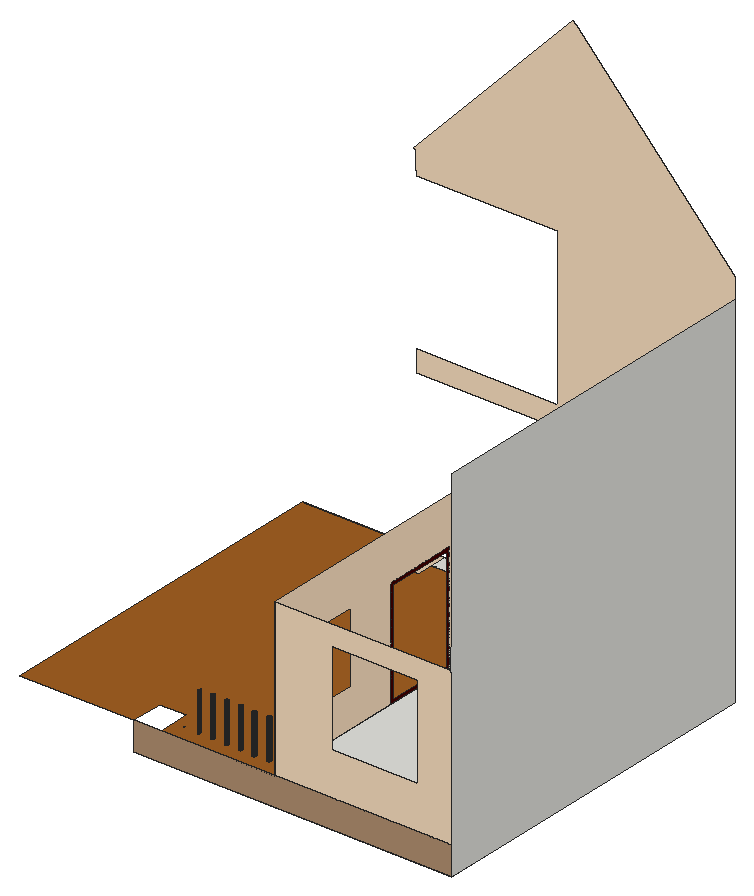
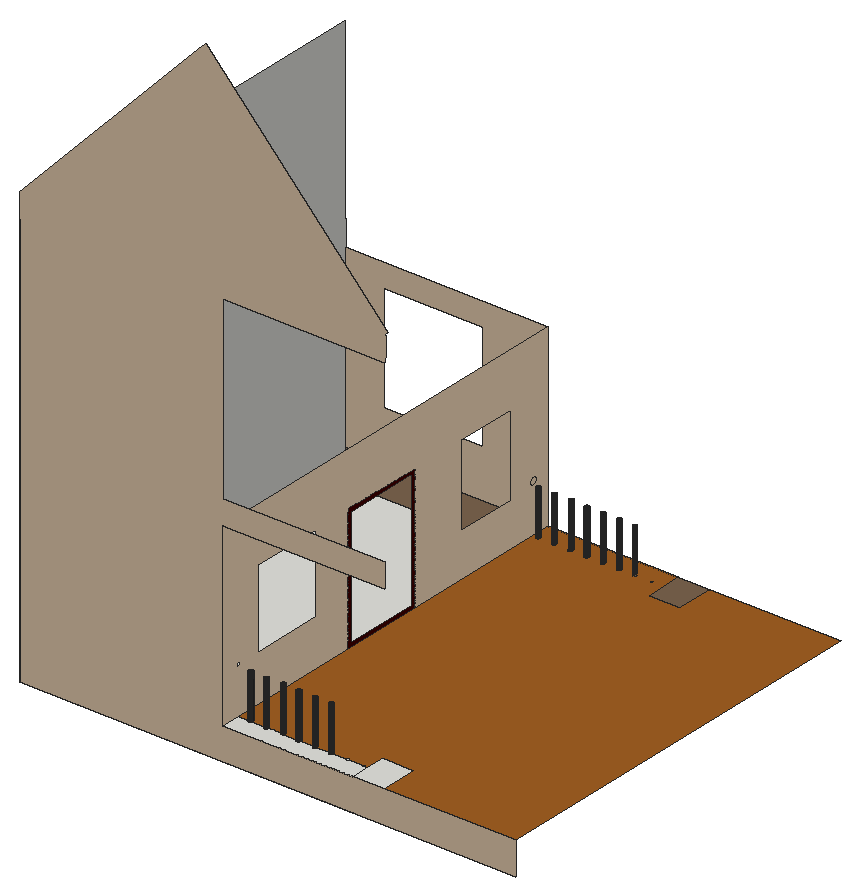
# SketchUp Ruby script. Lengths in inches.
U = 1.inch
M = Sketchup.active_model
def pt(a) = Geom::Point3d.new(a.map { |v| v * U })
def face(e, loops, mat)
  f = e.add_face(loops[0].map { |a| pt(a) })
  loops[1..].each { |l| e.add_face(l.map { |a| pt(a) }).erase! }
  f.material = f.back_material = mat if mat
  f
end
# faces: each face lists its corners as indices into pts; further lists are holes
def faces(e, pts, list, mat = nil) = list.each { |f| face(e, (f[0].is_a?(Array) ? f : [f]).map { |l| l.map { |i| pts[i] } }, mat) }
# xy, xz, yz: faces in a plane at the given z, y or x. An outline is a flat list of corners, or four numbers for a rectangle; further outlines are holes
def ring(l) = l.size == 4 ? [[l[0], l[1]], [l[2], l[1]], [l[2], l[3]], [l[0], l[3]]] : l.each_slice(2).to_a
def flat(e, list, mat, &to3) = list.each { |f| face(e, (f[0].is_a?(Array) ? f : [f]).map { |l| ring(l).map { |u, v| to3.(u, v) } }, mat) }
def xy(e, z, list, mat = nil) = flat(e, list, mat) { |x, y| [x, y, z] }
def xz(e, y, list, mat = nil) = flat(e, list, mat) { |x, z| [x, y, z] }
def yz(e, x, list, mat = nil) = flat(e, list, mat) { |y, z| [x, y, z] }
def lines(e, pts, list) = list.each { |a, b| e.add_line(pt(pts[a]), pt(pts[b])) }
# prism: a flat outline (further loops are holes) pulled along v
def prism(e, loops, v, mat = nil)
  f = face(e, loops, mat); d = Geom::Vector3d.new(v.map { |x| x * U })
  f.pushpull(f.normal.samedirection?(d) ? d.length : -d.length)
end
def box(e, o, s, mat = nil) = prism(e, [[o, [o[0] + s[0], o[1], o[2]], [o[0] + s[0], o[1] + s[1], o[2]], [o[0], o[1] + s[1], o[2]]]], [0, 0, s[2]], mat)
def at(x, y, z, deg = 0) = Geom::Transformation.translation(pt([x, y, z])) * Geom::Transformation.rotation(ORIGIN, Z_AXIS, deg.degrees)
def axes(o, x, y, z) = Geom::Transformation.new([*x, 0, *y, 0, *z, 0, *pt(o).to_a, 1])
def part(name) = M.definitions.add(name)
# library, detail: a bought-in or finely detailed component or shape, given as its bounding box
def library(name, o, s) = part(name).tap { |d| box(d.entities, o, s) }
def detail(e, o, s) = box(e.add_group.entities, o, s)
def put(e, d, t, mat = nil) = e.add_instance(d, t).tap { |i| i.material = mat if mat }
def group(e, t, mat = nil) = e.add_group.tap { |g| g.transformation = t; g.material = mat if mat }.entities
root = M.entities
M.materials.add("[0012_Bisque]").color = [255, 228, 196]
M.materials.add("[0022_Maroon]").color = [68, 0, 0]
M.materials.add("[0137_Black]").color = [45, 45, 45]
M.materials.add("[Stone Masonry Multi]").color = [182, 147, 116]
M.materials.add("[Wood Square Tile 02]").color = [160, 95, 34]
xy(root,0,[[240,84,732,684]])
xy(root,48,[[305.12,108.28,305.9,108.38,306.62,108.68,307.24,109.16,307.72,109.78,308.02,110.5,308.12,111.28,308.02,112.06,307.72,112.78,307.24,113.4,306.62,113.88,305.9,114.18,305.12,114.28,304.34,114.18,303.62,113.88,303,113.4,302.52,112.78,302.22,112.06,302.12,111.28,302.22,110.5,302.52,109.78,303,109.16,303.62,108.68,304.34,108.38],[329.12,108.28,329.9,108.38,330.62,108.68,331.24,109.16,331.72,109.78,332.02,110.5,332.12,111.28,332.02,112.06,331.72,112.78,331.24,113.4,330.62,113.88,329.9,114.18,329.12,114.28,328.34,114.18,327.62,113.88,327,113.4,326.52,112.78,326.22,112.06,326.12,111.28,326.22,110.5,326.52,109.78,327,109.16,327.62,108.68,328.34,108.38],[353.12,108.28,353.9,108.38,354.62,108.68,355.24,109.16,355.72,109.78,356.02,110.5,356.12,111.28,356.02,112.06,355.72,112.78,355.24,113.4,354.62,113.88,353.9,114.18,353.12,114.28,352.34,114.18,351.62,113.88,351,113.4,350.52,112.78,350.22,112.06,350.12,111.28,350.22,110.5,350.52,109.78,351,109.16,351.62,108.68,352.34,108.38],[377.12,108.28,377.9,108.38,378.62,108.68,379.24,109.16,379.72,109.78,380.02,110.5,379.72,111.23,379.24,111.85,378.62,112.33,377.9,112.625,377.12,112.73,376.34,112.625,375.62,112.33,375,111.85,374.52,111.23,374.22,110.5,374.52,109.78,375,109.16,375.62,108.68,376.34,108.38],[401.12,108.28,401.9,108.38,402.62,108.68,403.24,109.16,403.72,109.78,404.02,110.5,404.12,111.28,404.02,112.06,403.72,112.78,403.24,113.4,402.62,113.88,401.9,114.18,401.12,114.28,400.34,114.18,399.62,113.88,399,113.4,398.52,112.78,398.22,112.06,398.12,111.28,398.22,110.5,398.52,109.78,399,109.16,399.62,108.68,400.34,108.38],
  [425.12,108.28,425.9,108.38,426.62,108.68,427.24,109.16,427.54,109.88,427.64,110.66,427.54,111.4375,427.24,112.16,426.77,112.78,426.14,113.26,425.42,113.56,424.64,113.66,423.87,113.56,423.14,113.26,422.52,112.78,422.22,112.06,422.12,111.28,422.22,110.5,422.52,109.78,423,109.16,423.62,108.68,424.34,108.38],[449.12,108.28,449.9,108.38,450.62,108.68,451.24,109.16,451.72,109.78,452.02,110.5,452.12,111.28,452.02,112.06,451.72,112.78,451.24,113.4,450.62,113.88,449.9,114.18,449.12,114.28,448.34,114.18,447.62,113.88,447,113.4,446.52,112.78,446.22,112.06,446.12,111.28,446.22,110.5,446.52,109.78,447,109.16,447.62,108.68,448.34,108.38],[427.24,109.16,427.72,109.78,428.02,110.5,428.12,111.28,428.02,112.06,427.72,112.78,427.24,113.4,426.62,113.88,425.9,114.18,425.12,114.28,424.34,114.18,423.62,113.88,423,113.4,422.52,112.78,423.14,113.26,423.87,113.56,424.64,113.66,425.42,113.56,426.14,113.26,426.77,112.78,427.24,112.16,427.54,111.4375,427.64,110.66,427.54,109.88],[374.22,110.5,374.52,111.23,375,111.85,375.62,112.33,376.34,112.625,377.12,112.73,377.9,112.625,378.62,112.33,379.24,111.85,379.72,111.23,380.02,110.5,380.12,111.28,380.02,112.06,379.72,112.78,379.24,113.4,378.62,113.88,377.9,114.18,377.12,114.28,376.34,114.18,375.62,113.88,375,113.4,374.52,112.78,374.22,112.06,374.12,111.28],[366.01,652.17,366.79,652.27,367.51,652.57,368.13,653.04,368.61,653.67,368.91,654.39,369.01,655.17,368.91,655.94,368.61,656.67,368.57,656.72,363.45,656.72,363.41,656.67,363.11,655.94,363.01,655.17,363.11,654.39,363.41,653.67,363.89,653.04,364.51,652.57,365.23,652.27],
  [413.53,653.1,414.31,653.2,415.03,653.5,415.65,653.98,416.13,654.6,416.43,655.32,416.53,656.1,416.45,656.72,410.61,656.72,410.53,656.1,410.63,655.32,410.93,654.6,411.41,653.98,412.03,653.5,412.76,653.2],[294.01,653.72,294.79,653.82,295.51,654.12,296.13,654.6,296.61,655.22,296.91,655.94,297.01,656.72,291.01,656.72,291.11,655.94,291.41,655.22,291.89,654.6,292.51,654.12,293.23,653.82],[318.01,653.72,318.79,653.82,319.51,654.12,320.13,654.6,320.61,655.22,320.91,655.94,321.01,656.72,315.01,656.72,315.11,655.94,315.41,655.22,315.89,654.6,316.51,654.12,317.23,653.82],[342.01,653.72,342.79,653.82,343.51,654.12,344.13,654.6,344.61,655.22,344.91,655.94,345.01,656.72,339.01,656.72,339.11,655.94,339.41,655.22,339.89,654.6,340.51,654.12,341.23,653.82],[390.01,653.72,390.79,653.82,391.51,654.12,392.13,654.6,392.61,655.22,392.91,655.94,393.01,656.72,387.01,656.72,387.11,655.94,387.41,655.22,387.89,654.6,388.51,654.12,389.23,653.82],
  [240,656.72,243.01,656.72,243.11,657.5,243.41,658.22,243.89,658.84,244.51,659.32,245.23,659.62,246.01,659.72,246.79,659.62,247.51,659.32,248.13,658.84,248.61,658.22,248.91,657.5,249.01,656.72,267.01,656.72,267.11,657.5,267.41,658.22,267.89,658.84,268.51,659.32,269.23,659.62,270.01,659.72,270.79,659.62,271.51,659.32,272.13,658.84,272.61,658.22,272.91,657.5,273.01,656.72,291.01,656.72,291.11,657.5,291.41,658.22,291.89,658.84,292.51,659.32,293.23,659.62,294.01,659.72,294.79,659.62,295.51,659.32,296.13,658.84,296.61,658.22,296.91,657.5,297.01,656.72,315.01,656.72,315.11,657.5,315.41,658.22,315.89,658.84,316.51,659.32,317.23,659.62,318.01,659.72,318.79,659.62,319.51,659.32,320.13,658.84,320.61,658.22,320.91,657.5,321.01,656.72,339.01,656.72,339.11,657.5,339.41,658.22,339.89,658.84,340.51,659.32,341.23,659.62,342.01,659.72,342.79,659.62,343.51,659.32,344.13,658.84,344.61,658.22,344.91,657.5,345.01,656.72,363.45,656.72,363.89,657.29,364.51,657.76,365.23,658.0625,366.01,658.17,366.79,658.0625,367.51,657.76,368.13,657.29,368.57,656.72,387.01,656.72,387.11,657.5,387.41,658.22,387.89,658.84,388.51,659.32,389.23,659.62,390.01,659.72,390.79,659.62,391.51,659.32,392.13,658.84,392.61,658.22,392.91,657.5,393.01,656.72,410.61,656.72,410.63,656.875,410.93,657.6,411.41,658.22,412.03,658.7,412.76,659,413.53,659.1,414.31,659,415.03,658.7,415.65,658.22,416.13,657.6,416.43,656.875,416.45,656.72,432,656.72,432,684,240,684],[291.01,656.72,297.01,656.72,296.91,657.5,296.61,658.22,296.13,658.84,295.51,659.32,294.79,659.62,294.01,659.72,293.23,659.62,292.51,659.32,291.89,658.84,291.41,658.22,291.11,657.5],[315.01,656.72,321.01,656.72,320.91,657.5,320.61,658.22,320.13,658.84,319.51,659.32,318.79,659.62,318.01,659.72,317.23,659.62,316.51,659.32,315.89,658.84,315.41,658.22,315.11,657.5],[339.01,656.72,345.01,656.72,344.91,657.5,344.61,658.22,344.13,658.84,343.51,659.32,342.79,659.62,342.01,659.72,341.23,659.62,340.51,659.32,339.89,658.84,339.41,658.22,339.11,657.5],[363.45,656.72,368.57,656.72,368.13,657.29,367.51,657.76,366.79,658.0625,366.01,658.17,365.23,658.0625,364.51,657.76,363.89,657.29],
  [387.01,656.72,393.01,656.72,392.91,657.5,392.61,658.22,392.13,658.84,391.51,659.32,390.79,659.62,390.01,659.72,389.23,659.62,388.51,659.32,387.89,658.84,387.41,658.22,387.11,657.5],[410.61,656.72,416.45,656.72,416.43,656.875,416.13,657.6,415.65,658.22,415.03,658.7,414.31,659,413.53,659.1,412.76,659,412.03,658.7,411.41,658.22,410.93,657.6,410.63,656.875]])
xy(root,48,[[[0,84,193.3125,84,193.3125,138.5625,240,138.5625,240,84,432,84,432,656.72,416.45,656.72,416.53,656.1,416.43,655.32,416.13,654.6,415.65,653.98,415.03,653.5,414.31,653.2,413.53,653.1,412.76,653.2,412.03,653.5,411.41,653.98,410.93,654.6,410.63,655.32,410.53,656.1,410.61,656.72,393.01,656.72,392.91,655.94,392.61,655.22,392.13,654.6,391.51,654.12,390.79,653.82,390.01,653.72,389.23,653.82,388.51,654.12,387.89,654.6,387.41,655.22,387.11,655.94,387.01,656.72,368.57,656.72,368.61,656.67,368.91,655.94,369.01,655.17,368.91,654.39,368.61,653.67,368.13,653.04,367.51,652.57,366.79,652.27,366.01,652.17,365.23,652.27,364.51,652.57,363.89,653.04,363.41,653.67,363.11,654.39,363.01,655.17,363.11,655.94,363.41,656.67,363.45,656.72,345.01,656.72,344.91,655.94,344.61,655.22,344.13,654.6,343.51,654.12,342.79,653.82,342.01,653.72,341.23,653.82,340.51,654.12,339.89,654.6,339.41,655.22,339.11,655.94,339.01,656.72,321.01,656.72,320.91,655.94,320.61,655.22,320.13,654.6,319.51,654.12,318.79,653.82,318.01,653.72,317.23,653.82,316.51,654.12,315.89,654.6,315.41,655.22,315.11,655.94,315.01,656.72,297.01,656.72,296.91,655.94,296.61,655.22,296.13,654.6,295.51,654.12,294.79,653.82,294.01,653.72,293.23,653.82,292.51,654.12,291.89,654.6,291.41,655.22,291.11,655.94,291.01,656.72,273.01,656.72,272.91,655.94,272.61,655.22,272.13,654.6,271.51,654.12,270.79,653.82,270.01,653.72,269.23,653.82,268.51,654.12,267.89,654.6,267.41,655.22,267.11,655.94,267.01,656.72,249.01,656.72,248.91,655.94,248.61,655.22,248.13,654.6,247.51,654.12,246.79,653.82,246.01,653.72,245.23,653.82,244.51,654.12,243.89,654.6,243.41,655.22,243.11,655.94,243.01,656.72,240,656.72,240,629.4375,193.3125,629.4375,193.3125,684,0,684],[257.12,108.28,256.34,108.38,255.62,108.68,255,109.16,254.52,109.78,254.22,110.5,254.12,111.28,254.22,112.06,254.52,112.78,255,113.4,255.62,113.88,256.34,114.18,257.12,114.28,257.9,114.18,258.62,113.88,259.24,113.4,259.72,112.78,260.02,112.06,260.12,111.28,260.02,110.5,259.72,109.78,259.24,109.16,258.62,108.68,257.9,108.38],[425.12,108.28,424.34,108.38,423.62,108.68,423,109.16,422.52,109.78,422.22,110.5,422.12,111.28,422.22,112.06,422.52,112.78,423,113.4,423.62,113.88,424.34,114.18,425.12,114.28,425.9,114.18,426.62,113.88,427.24,113.4,427.72,112.78,428.02,112.06,428.12,111.28,428.02,110.5,427.72,109.78,427.24,109.16,426.62,108.68,425.9,108.38],[401.12,108.28,400.34,108.38,399.62,108.68,399,109.16,398.52,109.78,398.22,110.5,398.12,111.28,398.22,112.06,398.52,112.78,399,113.4,399.62,113.88,400.34,114.18,401.12,114.28,401.9,114.18,402.62,113.88,403.24,113.4,403.72,112.78,404.02,112.06,404.12,111.28,404.02,110.5,403.72,109.78,403.24,109.16,402.62,108.68,401.9,108.38],[377.12,108.28,376.34,108.38,375.62,108.68,375,109.16,374.52,109.78,374.22,110.5,374.12,111.28,374.22,112.06,374.52,112.78,375,113.4,375.62,113.88,376.34,114.18,377.12,114.28,377.9,114.18,378.62,113.88,379.24,113.4,379.72,112.78,380.02,112.06,380.12,111.28,380.02,110.5,379.72,109.78,379.24,109.16,378.62,108.68,377.9,108.38],[353.12,108.28,352.34,108.38,351.62,108.68,351,109.16,350.52,109.78,350.22,110.5,350.12,111.28,350.22,112.06,350.52,112.78,351,113.4,351.62,113.88,352.34,114.18,353.12,114.28,353.9,114.18,354.62,113.88,355.24,113.4,355.72,112.78,356.02,112.06,356.12,111.28,356.02,110.5,355.72,109.78,355.24,109.16,354.62,108.68,353.9,108.38],[329.12,108.28,328.34,108.38,327.62,108.68,327,109.16,326.52,109.78,326.22,110.5,326.12,111.28,326.22,112.06,326.52,112.78,327,113.4,327.62,113.88,328.34,114.18,329.12,114.28,329.9,114.18,330.62,113.88,331.24,113.4,331.72,112.78,332.02,112.06,332.12,111.28,332.02,110.5,331.72,109.78,331.24,109.16,330.62,108.68,329.9,108.38],[305.12,108.28,304.34,108.38,303.62,108.68,303,109.16,302.52,109.78,302.22,110.5,302.12,111.28,302.22,112.06,302.52,112.78,303,113.4,303.62,113.88,304.34,114.18,305.12,114.28,305.9,114.18,306.62,113.88,307.24,113.4,307.72,112.78,308.02,112.06,308.12,111.28,308.02,110.5,307.72,109.78,307.24,109.16,306.62,108.68,305.9,108.38],[281.12,108.28,280.34,108.38,279.62,108.68,279,109.16,278.52,109.78,278.22,110.5,278.12,111.28,278.22,112.06,278.52,112.78,279,113.4,279.62,113.88,280.34,114.18,281.12,114.28,281.9,114.18,282.62,113.88,283.24,113.4,283.72,112.78,284.02,112.06,284.12,111.28,284.02,110.5,283.72,109.78,283.24,109.16,282.62,108.68,281.9,108.38]]],"[Wood Square Tile 02]")
xz(root,84,[[[432,48,732,312],[528.3,119.9,674.74,278.46]]],"[0012_Bisque]")
xz(root,84,[[193.3125,0,732,48]],"[Stone Masonry Multi]")
xz(root,684,[[0,0,0,48,432,48,432,312,193.3125,312,193.3125,348,432,348,432,612,193.3125,612,193.3125,619.2,191.3125,619.2,191.3125,648,193.3125,648,188.41,652.59,457.75,940.59,462.66,936,732,648,732,0]],"[0012_Bisque]")
yz(root,432,[[[84,48,84,312,684,312,684,48,453.05,48,453.05,232.5,329.93,232.5,329.93,48],[513.28,116.55,620.09,231.74],[153.23,112.5,244.92,232.5],[111.28,114,111.91,114.03,112.53,114.13,113.14,114.29,113.72,114.52,114.28,114.8,114.81,115.15,115.3,115.54,115.74,115.99,116.14,116.47,116.48,117,116.76,117.56,116.99,118.15,117.15,118.75,117.25,119.37,117.28,120,117.25,120.63,117.15,121.25,116.99,121.85,116.76,122.44,116.48,123,116.14,123.53,115.74,124.01,115.3,124.46,114.81,124.85,114.28,125.2,113.72,125.48,113.14,125.71,112.53,125.87,111.91,125.97,111.28,126,110.65,125.97,110.03,125.87,109.43,125.71,108.84,125.48,108.28,125.2,107.75,124.85,107.27,124.46,106.82,124.01,106.43,123.53,106.09,123,105.8,122.44,105.57,121.85,105.41,121.25,105.3125,120.63,105.28,120,105.3125,119.37,105.41,118.75,105.57,118.15,105.8,117.56,106.09,117,106.43,116.47,106.82,115.99,107.27,115.54,107.75,115.15,108.28,114.8,108.84,114.52,109.43,114.29,110.03,114.13,110.65,114.03],[655.94,113.61,656.72,113.71,657.44,114.01,658.0625,114.49,658.54,115.11,658.84,115.83,658.94,116.61,658.84,117.39,658.54,118.11,658.0625,118.73,657.44,119.21,656.72,119.51,655.94,119.61,655.17,119.51,654.44,119.21,653.82,118.73,653.34,118.11,653.04,117.39,652.94,116.61,653.04,115.83,653.34,115.11,653.82,114.49,654.44,114.01,655.17,113.71]]],"[0012_Bisque]")
yz(root,432,[[[329.93,48,453.05,232.5],[334.98,53.06,447.99,227.44]]],"[0022_Maroon]")
yz(root,732,[[84,0,684,0,684,612,84,612,84,348,82,348,82,312,84,312]])
p = [[376.34,106.83,48],[377.12,106.73,48],[377.12,106.73,113.8],[376.34,106.83,113.8],[377.9,106.83,48],[377.9,106.83,113.8],
  [375.62,107.13,48],[375.62,107.13,113.8],[378.62,107.13,48],[378.62,107.13,113.8],[375,107.61,48],[375,107.61,113.8],
  [379.24,107.61,48],[379.24,107.61,113.8],[374.52,108.23,48],[374.52,108.23,113.8],[379.72,108.23,48],[379.72,108.23,113.8],
  [423.87,107.76,48],[424.64,107.66,48],[424.64,107.66,113.8],[423.87,107.76,113.8],[425.42,107.76,48],[425.42,107.76,113.8],
  [423.14,108.0625,48],[423.14,108.0625,113.8],[426.14,108.0625,48],[426.14,108.0625,113.8],[422.52,108.54,48],[422.52,108.54,113.8],
  [426.77,108.54,48],[426.77,108.54,113.8],[374.22,108.95,48],[374.22,108.95,113.8],[380.02,108.95,48],[380.02,108.95,113.8],
  [304.34,108.38,48],[305.12,108.28,48],[305.12,108.28,113.8],[304.34,108.38,113.8],[305.9,108.38,48],[305.9,108.38,113.8],
  [328.34,108.38,48],[329.12,108.28,48],[329.12,108.28,113.8],[328.34,108.38,113.8],[329.9,108.38,48],[329.9,108.38,113.8],
  [352.34,108.38,48],[353.12,108.28,48],[353.12,108.28,113.8],[352.34,108.38,113.8],[353.9,108.38,48],[353.9,108.38,113.8],
  [400.34,108.38,48],[401.12,108.28,48],[401.12,108.28,113.8],[400.34,108.38,113.8],[401.9,108.38,48],[401.9,108.38,113.8],
  [281.9,108.38,48],[282.62,108.68,48],[282.62,108.68,113.8],[281.9,108.38,113.8],[303.62,108.68,48],[303.62,108.68,113.8],
  [306.62,108.68,48],[306.62,108.68,113.8],[327.62,108.68,48],[327.62,108.68,113.8],[330.62,108.68,48],[330.62,108.68,113.8],
  [351.62,108.68,48],[351.62,108.68,113.8],[354.62,108.68,48],[354.62,108.68,113.8],[399.62,108.68,48],[399.62,108.68,113.8],
  [402.62,108.68,48],[402.62,108.68,113.8],[422.05,109.16,48],[422.05,109.16,113.8],[427.24,109.16,48],[427.24,109.16,113.8],
  [283.24,109.16,48],[283.24,109.16,113.8],[303,109.16,48],[303,109.16,113.8],[307.24,109.16,48],[307.24,109.16,113.8],
  [327,109.16,48],[327,109.16,113.8],[331.24,109.16,48],[331.24,109.16,113.8],[351,109.16,48],[351,109.16,113.8],
  [355.24,109.16,48],[355.24,109.16,113.8],[399,109.16,48],[399,109.16,113.8],[403.24,109.16,48],[403.24,109.16,113.8],
  [374.12,109.73,48],[374.12,109.73,113.8],[380.12,109.73,48],[380.12,109.73,113.8],[283.72,109.78,48],[283.72,109.78,113.8],
  [302.52,109.78,48],[302.52,109.78,113.8],[307.72,109.78,48],[307.72,109.78,113.8],[326.52,109.78,48],[326.52,109.78,113.8],
  [331.72,109.78,48],[331.72,109.78,113.8],[350.52,109.78,48],[350.52,109.78,113.8],[355.72,109.78,48],[355.72,109.78,113.8],
  [398.52,109.78,48],[398.52,109.78,113.8],[403.72,109.78,48],[403.72,109.78,113.8],[421.75,109.88,48],[421.75,109.88,113.8],
  [427.54,109.88,48],[427.54,109.88,113.8],[374.22,110.5,48],[374.22,110.5,113.8],[380.02,110.5,48],[380.02,110.5,113.8],
  [284.02,110.5,48],[284.02,110.5,113.8],[302.22,110.5,48],[302.22,110.5,113.8],[308.02,110.5,48],[308.02,110.5,113.8],
  [326.22,110.5,48],[326.22,110.5,113.8],[332.02,110.5,48],[332.02,110.5,113.8],[350.22,110.5,48],[350.22,110.5,113.8],
  [356.02,110.5,48],[356.02,110.5,113.8],[398.22,110.5,48],[398.22,110.5,113.8],[404.02,110.5,48],[404.02,110.5,113.8],
  [421.64,110.66,48],[421.64,110.66,113.8],[427.64,110.66,48],[427.64,110.66,113.8],[284.12,111.28,48],[284.12,111.28,113.8],
  [302.12,111.28,48],[302.12,111.28,113.8],[308.12,111.28,48],[308.12,111.28,113.8],[326.12,111.28,48],[326.12,111.28,113.8],
  [332.12,111.28,48],[332.12,111.28,113.8],[350.12,111.28,48],[350.12,111.28,113.8],[356.12,111.28,48],[356.12,111.28,113.8],
  [374.52,111.23,48],[374.52,111.23,113.8],[379.72,111.23,48],[379.72,111.23,113.8],[398.12,111.28,48],[398.12,111.28,113.8],
  [404.12,111.28,48],[404.12,111.28,113.8],[421.75,111.4375,48],[421.75,111.4375,113.8],[427.54,111.4375,48],[427.54,111.4375,113.8],
  [375,111.85,48],[375,111.85,113.8],[379.24,111.85,48],[379.24,111.85,113.8],[284.02,112.06,48],[284.02,112.06,113.8],
  [302.22,112.06,48],[302.22,112.06,113.8],[308.02,112.06,48],[308.02,112.06,113.8],[326.22,112.06,48],[326.22,112.06,113.8],
  [332.02,112.06,48],[332.02,112.06,113.8],[350.22,112.06,48],[350.22,112.06,113.8],[356.02,112.06,48],[356.02,112.06,113.8],
  [398.22,112.06,48],[398.22,112.06,113.8],[404.02,112.06,48],[404.02,112.06,113.8],[422.05,112.16,48],[422.05,112.16,113.8],
  [427.24,112.16,48],[427.24,112.16,113.8],[375.62,112.33,48],[375.62,112.33,113.8],[378.62,112.33,48],[378.62,112.33,113.8],
  [283.72,112.78,48],[283.72,112.78,113.8],[302.52,112.78,48],[302.52,112.78,113.8],[307.72,112.78,48],[307.72,112.78,113.8],
  [326.52,112.78,48],[326.52,112.78,113.8],[331.72,112.78,48],[331.72,112.78,113.8],[350.52,112.78,48],[350.52,112.78,113.8],
  [355.72,112.78,48],[355.72,112.78,113.8],[398.52,112.78,48],[398.52,112.78,113.8],[403.72,112.78,48],[403.72,112.78,113.8],
  [422.52,112.78,48],[422.52,112.78,113.8],[426.77,112.78,48],[426.77,112.78,113.8],[376.34,112.625,48],[376.34,112.625,113.8],
  [377.9,112.625,48],[377.9,112.625,113.8],[377.12,112.73,48],[377.12,112.73,113.8],[283.24,113.4,48],[283.24,113.4,113.8],
  [303,113.4,48],[303,113.4,113.8],[307.24,113.4,48],[307.24,113.4,113.8],[327,113.4,48],[327,113.4,113.8],
  [331.24,113.4,48],[331.24,113.4,113.8],[351,113.4,48],[351,113.4,113.8],[355.24,113.4,48],[355.24,113.4,113.8],
  [399,113.4,48],[399,113.4,113.8],[403.24,113.4,48],[403.24,113.4,113.8],[423.14,113.26,48],[423.14,113.26,113.8],
  [426.14,113.26,48],[426.14,113.26,113.8],[423.87,113.56,48],[423.87,113.56,113.8],[425.42,113.56,48],[425.42,113.56,113.8],
  [282.62,113.88,48],[282.62,113.88,113.8],[303.62,113.88,48],[303.62,113.88,113.8],[306.62,113.88,48],[306.62,113.88,113.8],
  [327.62,113.88,48],[327.62,113.88,113.8],[330.62,113.88,48],[330.62,113.88,113.8],[351.62,113.88,48],[351.62,113.88,113.8],
  [354.62,113.88,48],[354.62,113.88,113.8],[399.62,113.88,48],[399.62,113.88,113.8],[402.62,113.88,48],[402.62,113.88,113.8],
  [424.64,113.66,48],[424.64,113.66,113.8],[304.34,114.18,48],[304.34,114.18,113.8],[305.9,114.18,48],[305.9,114.18,113.8],
  [328.34,114.18,48],[328.34,114.18,113.8],[329.9,114.18,48],[329.9,114.18,113.8],[352.34,114.18,48],[352.34,114.18,113.8],
  [353.9,114.18,48],[353.9,114.18,113.8],[400.34,114.18,48],[400.34,114.18,113.8],[401.9,114.18,48],[401.9,114.18,113.8],
  [305.12,114.28,48],[305.12,114.28,113.8],[329.12,114.28,48],[329.12,114.28,113.8],[353.12,114.28,48],[353.12,114.28,113.8],
  [401.12,114.28,48],[401.12,114.28,113.8],[365.23,652.27,48],[366.01,652.17,48],[366.01,652.17,113.8],[365.23,652.27,113.8],
  [366.79,652.27,48],[366.79,652.27,113.8],[364.51,652.57,48],[364.51,652.57,113.8],[367.51,652.57,48],[367.51,652.57,113.8],
  [363.89,653.04,48],[363.89,653.04,113.8],[368.13,653.04,48],[368.13,653.04,113.8],[363.41,653.67,48],[363.41,653.67,113.8],
  [368.61,653.67,48],[368.61,653.67,113.8],[412.76,653.2,48],[413.53,653.1,48],[413.53,653.1,113.8],[412.76,653.2,113.8],
  [414.31,653.2,48],[414.31,653.2,113.8],[412.03,653.5,48],[412.03,653.5,113.8],[415.03,653.5,48],[415.03,653.5,113.8],
  [411.41,653.98,48],[411.41,653.98,113.8],[415.65,653.98,48],[415.65,653.98,113.8],[293.23,653.82,48],[294.01,653.72,48],
  [294.01,653.72,113.8],[293.23,653.82,113.8],[294.79,653.82,48],[294.79,653.82,113.8],[317.23,653.82,48],[318.01,653.72,48],
  [318.01,653.72,113.8],[317.23,653.82,113.8],[318.79,653.82,48],[318.79,653.82,113.8],[341.23,653.82,48],[342.01,653.72,48],
  [342.01,653.72,113.8],[341.23,653.82,113.8],[342.79,653.82,48],[342.79,653.82,113.8],[363.11,654.39,48],[363.11,654.39,113.8],
  [368.91,654.39,48],[368.91,654.39,113.8],[389.23,653.82,48],[390.01,653.72,48],[390.01,653.72,113.8],[389.23,653.82,113.8],
  [390.79,653.82,48],[390.79,653.82,113.8],[292.51,654.12,48],[292.51,654.12,113.8],[295.51,654.12,48],[295.51,654.12,113.8],
  [316.51,654.12,48],[316.51,654.12,113.8],[319.51,654.12,48],[319.51,654.12,113.8],[340.51,654.12,48],[340.51,654.12,113.8],
  [343.51,654.12,48],[343.51,654.12,113.8],[388.51,654.12,48],[388.51,654.12,113.8],[391.51,654.12,48],[391.51,654.12,113.8],
  [410.93,654.6,48],[410.93,654.6,113.8],[416.13,654.6,48],[416.13,654.6,113.8],[291.89,654.6,48],[291.89,654.6,113.8],
  [296.13,654.6,48],[296.13,654.6,113.8],[315.89,654.6,48],[315.89,654.6,113.8],[320.13,654.6,48],[320.13,654.6,113.8],
  [339.89,654.6,48],[339.89,654.6,113.8],[344.13,654.6,48],[344.13,654.6,113.8],[387.89,654.6,48],[387.89,654.6,113.8],
  [392.13,654.6,48],[392.13,654.6,113.8],[363.01,655.17,48],[363.01,655.17,113.8],[363.01,655.17,113.71],[369.01,655.17,48],
  [369.01,655.17,113.71],[369.01,655.17,113.8],[291.41,655.22,48],[291.41,655.22,113.8],[296.61,655.22,48],[296.61,655.22,113.8],
  [315.41,655.22,48],[315.41,655.22,113.8],[320.61,655.22,48],[320.61,655.22,113.8],[339.41,655.22,48],[339.41,655.22,113.8],
  [344.61,655.22,48],[344.61,655.22,113.8],[387.41,655.22,48],[387.41,655.22,113.8],[392.61,655.22,48],[392.61,655.22,113.8],
  [410.63,655.32,48],[410.63,655.32,113.8],[416.43,655.32,48],[416.43,655.32,113.8],[291.11,655.94,48],[291.11,655.94,113.8],
  [291.11,655.94,113.61],[296.91,655.94,48],[296.91,655.94,113.61],[296.91,655.94,113.8],[315.11,655.94,48],[315.11,655.94,113.8],
  [315.11,655.94,113.61],[320.91,655.94,48],[320.91,655.94,113.61],[320.91,655.94,113.8],[339.11,655.94,48],[339.11,655.94,113.8],
  [339.11,655.94,113.61],[344.91,655.94,48],[344.91,655.94,113.61],[344.91,655.94,113.8],[363.11,655.94,48],[363.11,655.94,113.8],
  [363.11,655.94,113.61],[368.91,655.94,48],[368.91,655.94,113.61],[368.91,655.94,113.8],[387.11,655.94,48],[387.11,655.94,113.8],
  [387.11,655.94,113.61],[392.91,655.94,48],[392.91,655.94,113.61],[392.91,655.94,113.8],[410.53,656.1,48],[410.53,656.1,113.8],
  [416.53,656.1,48],[416.53,656.1,113.8],[291.01,656.72,48],[291.01,656.72,113.8],[291.01,656.72,113.71],[297.01,656.72,48],
  [297.01,656.72,113.71],[297.01,656.72,113.8],[315.01,656.72,48],[315.01,656.72,113.8],[315.01,656.72,113.71],[321.01,656.72,48],
  [321.01,656.72,113.71],[321.01,656.72,113.8],[339.01,656.72,48],[339.01,656.72,113.8],[339.01,656.72,113.71],[345.01,656.72,48],
  [345.01,656.72,113.71],[345.01,656.72,113.8],[363.41,656.67,48],[363.41,656.67,113.8],[368.61,656.67,48],[368.61,656.67,113.8],
  [387.01,656.72,48],[387.01,656.72,113.8],[387.01,656.72,113.71],[393.01,656.72,48],[393.01,656.72,113.71],[393.01,656.72,113.8],
  [410.63,656.875,48],[410.61,656.72,48],[410.63,656.875,113.8],[416.45,656.72,48],[416.43,656.875,48],[416.43,656.875,113.8],
  [291.11,657.5,48],[291.11,657.5,113.8],[296.91,657.5,48],[296.91,657.5,113.8],[315.11,657.5,48],[315.11,657.5,113.8],
  [320.91,657.5,48],[320.91,657.5,113.8],[339.11,657.5,48],[339.11,657.5,113.8],[344.91,657.5,48],[344.91,657.5,113.8],
  [363.89,657.29,48],[363.45,656.72,48],[363.89,657.29,113.8],[368.57,656.72,48],[368.13,657.29,48],[368.13,657.29,113.8],
  [387.11,657.5,48],[387.11,657.5,113.8],[392.91,657.5,48],[392.91,657.5,113.8],[410.93,657.6,48],[410.93,657.6,113.8],
  [416.13,657.6,48],[416.13,657.6,113.8],[364.51,657.76,48],[364.51,657.76,113.8],[367.51,657.76,48],[367.51,657.76,113.8],
  [291.41,658.22,48],[291.41,658.22,113.8],[296.61,658.22,48],[296.61,658.22,113.8],[315.41,658.22,48],[315.41,658.22,113.8],
  [320.61,658.22,48],[320.61,658.22,113.8],[339.41,658.22,48],[339.41,658.22,113.8],[344.61,658.22,48],[344.61,658.22,113.8],
  [387.41,658.22,48],[387.41,658.22,113.8],[392.61,658.22,48],[392.61,658.22,113.8],[411.41,658.22,48],[411.41,658.22,113.8],
  [415.65,658.22,48],[415.65,658.22,113.8],[365.23,658.0625,48],[365.23,658.0625,113.8],[366.79,658.0625,48],[366.79,658.0625,113.8],
  [366.01,658.17,48],[366.01,658.17,113.8],[291.89,658.84,48],[291.89,658.84,113.8],[296.13,658.84,48],[296.13,658.84,113.8],
  [315.89,658.84,48],[315.89,658.84,113.8],[320.13,658.84,48],[320.13,658.84,113.8],[339.89,658.84,48],[339.89,658.84,113.8],
  [344.13,658.84,48],[344.13,658.84,113.8],[387.89,658.84,48],[387.89,658.84,113.8],[392.13,658.84,48],[392.13,658.84,113.8],
  [412.03,658.7,48],[412.03,658.7,113.8],[415.03,658.7,48],[415.03,658.7,113.8],[412.76,659,48],[412.76,659,113.8],
  [414.31,659,48],[414.31,659,113.8],[292.51,659.32,48],[292.51,659.32,113.8],[295.51,659.32,48],[295.51,659.32,113.8],
  [316.51,659.32,48],[316.51,659.32,113.8],[319.51,659.32,48],[319.51,659.32,113.8],[340.51,659.32,48],[340.51,659.32,113.8],
  [343.51,659.32,48],[343.51,659.32,113.8],[388.51,659.32,48],[388.51,659.32,113.8],[391.51,659.32,48],[391.51,659.32,113.8],
  [413.53,659.1,48],[413.53,659.1,113.8],[293.23,659.62,48],[293.23,659.62,113.8],[294.79,659.62,48],[294.79,659.62,113.8],
  [317.23,659.62,48],[317.23,659.62,113.8],[318.79,659.62,48],[318.79,659.62,113.8],[341.23,659.62,48],[341.23,659.62,113.8],
  [342.79,659.62,48],[342.79,659.62,113.8],[389.23,659.62,48],[389.23,659.62,113.8],[390.79,659.62,48],[390.79,659.62,113.8],
  [294.01,659.72,48],[294.01,659.72,113.8],[318.01,659.72,48],[318.01,659.72,113.8],[342.01,659.72,48],[342.01,659.72,113.8],
  [390.01,659.72,48],[390.01,659.72,113.8],[305.12,111.28,48],[305.12,111.28,113.8],[329.12,111.28,48],[329.12,111.28,114],
  [353.12,111.28,48],[353.12,111.28,114],[377.12,111.28,48],[377.12,111.28,114],[401.12,111.28,48],[401.12,111.28,114],
  [425.12,111.28,48],[425.12,111.28,114],[366.01,656.72,48],[366.01,656.72,113.71]]
faces(root,p,[[0,1,2,3],[1,4,5,2],[6,0,3,7],[4,8,9,5],[10,6,7,11],[8,12,13,9],[14,10,11,15],[12,16,17,13],
  [18,19,20,21],[19,22,23,20],[24,18,21,25],[22,26,27,23],[28,24,25,29],[26,30,31,27],[32,14,15,33],[16,34,35,17],
  [36,37,38,39],[37,40,41,38],[42,43,44,45],[43,46,47,44],[48,49,50,51],[49,52,53,50],[54,55,56,57],[55,58,59,56],
  [60,61,62,63],[64,36,39,65],[40,66,67,41],[68,42,45,69],[46,70,71,47],[72,48,51,73],[52,74,75,53],[76,54,57,77],
  [58,78,79,59],[80,28,29,81],[30,82,83,31],[61,84,85,62],[86,64,65,87],[66,88,89,67],[90,68,69,91],[70,92,93,71],
  [94,72,73,95],[74,96,97,75],[98,76,77,99],[78,100,101,79],[102,32,33,103],[34,104,105,35],[84,106,107,85],[108,86,87,109],
  [88,110,111,89],[112,90,91,113],[92,114,115,93],[116,94,95,117],[96,118,119,97],[120,98,99,121],[100,122,123,101],[124,80,81,125],
  [82,126,127,83],[128,102,103,129],[104,130,131,105],[106,132,133,107],[134,108,109,135],[110,136,137,111],[138,112,113,139],[114,140,141,115],
  [142,116,117,143],[118,144,145,119],[146,120,121,147],[122,148,149,123],[150,124,125,151],[126,152,153,127],[132,154,155,133],[156,134,135,157],
  [136,158,159,137],[160,138,139,161],[140,162,163,141],[164,142,143,165],[144,166,167,145],[168,128,129,169],[130,170,171,131],[172,146,147,173],
  [148,174,175,149],[176,150,151,177],[152,178,179,153],[180,168,169,181],[170,182,183,171],[154,184,185,155],[186,156,157,187],[158,188,189,159],
  [190,160,161,191],[162,192,193,163],[194,164,165,195],[166,196,197,167],[198,172,173,199],[174,200,201,175],[202,176,177,203],[178,204,205,179],
  [206,180,181,207],[182,208,209,183],[184,210,211,185],[212,186,187,213],[188,214,215,189],[216,190,191,217],[192,218,219,193],[220,194,195,221],
  [196,222,223,197],[224,198,199,225],[200,226,227,201],[228,202,203,229],[204,230,231,205],[232,206,207,233],[208,234,235,209],[236,232,233,237],
  [234,236,237,235],[210,238,239,211],[240,212,213,241],[214,242,243,215],[244,216,217,245],[218,246,247,219],[248,220,221,249],[222,250,251,223],
  [252,224,225,253],[226,254,255,227],[256,228,229,257],[230,258,259,231],[260,256,257,261],[258,262,263,259],[238,264,265,239],[266,240,241,267],
  [242,268,269,243],[270,244,245,271],[246,272,273,247],[274,248,249,275],[250,276,277,251],[278,252,253,279],[254,280,281,255],[282,260,261,283],
  [262,282,283,263],[284,266,267,285],[268,286,287,269],[288,270,271,289],[272,290,291,273],[292,274,275,293],[276,294,295,277],[296,278,279,297],
  [280,298,299,281],[300,284,285,301],[286,300,301,287],[302,288,289,303],[290,302,303,291],[304,292,293,305],[294,304,305,295],[306,296,297,307],
  [298,306,307,299],[308,309,310,311],[309,312,313,310],[314,308,311,315],[312,316,317,313],[318,314,315,319],[316,320,321,317],[322,318,319,323],
  [320,324,325,321],[326,327,328,329],[327,330,331,328],[332,326,329,333],[330,334,335,331],[336,332,333,337],[334,338,339,335],[340,341,342,343],
  [341,344,345,342],[346,347,348,349],[347,350,351,348],[352,353,354,355],[353,356,357,354],[358,322,323,359],[324,360,361,325],[362,363,364,365],
  [363,366,367,364],[368,340,343,369],[344,370,371,345],[372,346,349,373],[350,374,375,351],[376,352,355,377],[356,378,379,357],[380,362,365,381],
  [366,382,383,367],[384,336,337,385],[338,386,387,339],[388,368,369,389],[370,390,391,371],[392,372,373,393],[374,394,395,375],[396,376,377,397],
  [378,398,399,379],[400,380,381,401],[382,402,403,383],[404,358,359,405,406],[360,407,408,409,361],[410,388,389,411],[390,412,413,391],[414,392,393,415],
  [394,416,417,395],[418,396,397,419],[398,420,421,399],[422,400,401,423],[402,424,425,403],[426,384,385,427],[386,428,429,387],[430,410,411,431,432],
  [412,433,434,435,413],[436,414,415,437,438],[416,439,440,441,417],[442,418,419,443,444],[420,445,446,447,421],[448,404,406,405,449,450],[407,451,452,453,409,408],[454,422,423,455,456],
  [424,457,458,459,425],[460,426,427,461],[428,462,463,429],[464,430,432,431,465,466],[433,467,468,469,435,434],[470,436,438,437,471,472],[439,473,474,475,441,440],[476,442,444,443,477,478],
  [445,479,480,481,447,446],[482,448,450,449,483],[451,484,485,453,452],[486,454,456,455,487,488],[457,489,490,491,459,458],[492,493,460,461,494],[462,495,496,497,463],[498,464,466,465,499],
  [467,500,501,469,468],[502,470,472,471,503],[473,504,505,475,474],[506,476,478,477,507],[479,508,509,481,480],[510,511,482,483,512],[484,513,514,515,485],[516,486,488,487,517],
  [489,518,519,491,490],[520,492,494,521],[496,522,523,497],[524,510,512,525],[514,526,527,515],[528,498,499,529],[500,530,531,501],[532,502,503,533],
  [504,534,535,505],[536,506,507,537],[508,538,539,509],[540,516,517,541],[518,542,543,519],[544,520,521,545],[522,546,547,523],[548,524,525,549],
  [526,550,551,527],[552,548,549,553],[550,552,553,551],[554,528,529,555],[530,556,557,531],[558,532,533,559],[534,560,561,535],[562,536,537,563],
  [538,564,565,539],[566,540,541,567],[542,568,569,543],[570,544,545,571],[546,572,573,547],[574,570,571,575],[572,576,577,573],[578,554,555,579],
  [556,580,581,557],[582,558,559,583],[560,584,585,561],[586,562,563,587],[564,588,589,565],[590,566,567,591],[568,592,593,569],[594,574,575,595],
  [576,594,595,577],[596,578,579,597],[580,598,599,581],[600,582,583,601],[584,602,603,585],[604,586,587,605],[588,606,607,589],[608,590,591,609],
  [592,610,611,593],[612,596,597,613],[598,612,613,599],[614,600,601,615],[602,614,615,603],[616,604,605,617],[606,616,617,607],[618,608,609,619],
  [610,618,619,611]],"[0137_Black]")
lines(root,p,[[620,621],[622,623],[624,625],[626,627],[628,629],[630,631],[632,633]])
